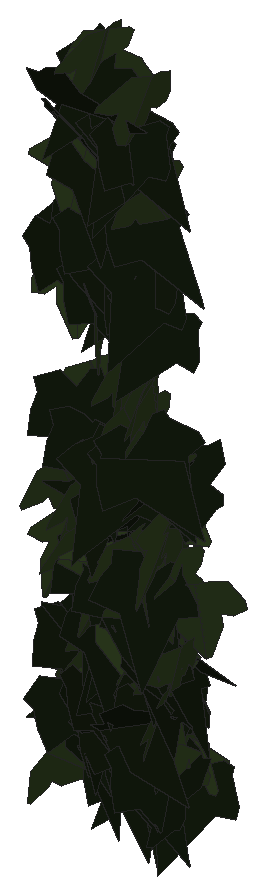
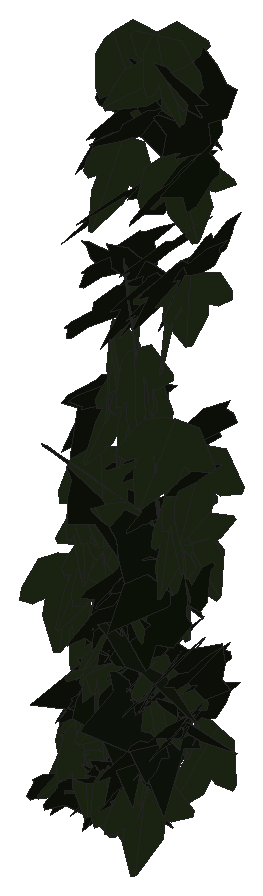
# SketchUp Ruby script. Lengths in inches.
U = 1.inch
M = Sketchup.active_model
def pt(a) = Geom::Point3d.new(a.map { |v| v * U })
def face(e, loops, mat)
  f = e.add_face(loops[0].map { |a| pt(a) })
  loops[1..].each { |l| e.add_face(l.map { |a| pt(a) }).erase! }
  f.material = f.back_material = mat if mat
  f
end
# faces: each face lists its corners as indices into pts; further lists are holes
def faces(e, pts, list, mat = nil) = list.each { |f| face(e, (f[0].is_a?(Array) ? f : [f]).map { |l| l.map { |i| pts[i] } }, mat) }
# xy, xz, yz: faces in a plane at the given z, y or x. An outline is a flat list of corners, or four numbers for a rectangle; further outlines are holes
def ring(l) = l.size == 4 ? [[l[0], l[1]], [l[2], l[1]], [l[2], l[3]], [l[0], l[3]]] : l.each_slice(2).to_a
def flat(e, list, mat, &to3) = list.each { |f| face(e, (f[0].is_a?(Array) ? f : [f]).map { |l| ring(l).map { |u, v| to3.(u, v) } }, mat) }
def xy(e, z, list, mat = nil) = flat(e, list, mat) { |x, y| [x, y, z] }
def xz(e, y, list, mat = nil) = flat(e, list, mat) { |x, z| [x, y, z] }
def yz(e, x, list, mat = nil) = flat(e, list, mat) { |y, z| [x, y, z] }
def lines(e, pts, list) = list.each { |a, b| e.add_line(pt(pts[a]), pt(pts[b])) }
# prism: a flat outline (further loops are holes) pulled along v
def prism(e, loops, v, mat = nil)
  f = face(e, loops, mat); d = Geom::Vector3d.new(v.map { |x| x * U })
  f.pushpull(f.normal.samedirection?(d) ? d.length : -d.length)
end
def box(e, o, s, mat = nil) = prism(e, [[o, [o[0] + s[0], o[1], o[2]], [o[0] + s[0], o[1] + s[1], o[2]], [o[0], o[1] + s[1], o[2]]]], [0, 0, s[2]], mat)
def at(x, y, z, deg = 0) = Geom::Transformation.translation(pt([x, y, z])) * Geom::Transformation.rotation(ORIGIN, Z_AXIS, deg.degrees)
def axes(o, x, y, z) = Geom::Transformation.new([*x, 0, *y, 0, *z, 0, *pt(o).to_a, 1])
def part(name) = M.definitions.add(name)
# library, detail: a bought-in or finely detailed component or shape, given as its bounding box
def library(name, o, s) = part(name).tap { |d| box(d.entities, o, s) }
def detail(e, o, s) = box(e.add_group.entities, o, s)
def put(e, d, t, mat = nil) = e.add_instance(d, t).tap { |i| i.material = mat if mat }
def group(e, t, mat = nil) = e.add_group.tap { |g| g.transformation = t; g.material = mat if mat }.entities
root = M.entities
M.materials.add("efeu1").color = [18, 25, 13]
M.materials.add("efeu2").color = [43, 57, 29]
c1 = part("ivyleaf_10")
p = [[0,0.5,-0.03],[-0.0625,2.02,-0.43],[-0.19,2.01,-0.46],[-0.54,1.05,-0.29],[-0.52,0.625,-0.18],[-0.83,0.76,-0.28],
  [-1.16,0.64,-0.33],[-1.15,0.33,-0.24],[-0.77,-0.39,0.02],[-0.3,-0.51,0.16],[0.04,-0.48,0.23],[-0.02,2.01,-0.4375],
  [-0.06,2.01,-0.43],[0.04,-0.49,0.23],[0.67,-0.49,0.14],[1.38,0.36,-0.2],[1.375,0.51,-0.24],[0.81,0.65,-0.19],
  [0.62,0.59,-0.15],[0.6,1.09,-0.28],[0.5,1.23,-0.31]]
faces(c1.entities,p,[[0,1,2,3,4,5,6,7,8,9,10],[11,12,0,13,14,15,16,17,18,19,20]],"efeu2")
c2 = part("ivyleaf_9")
p = [[1.54,2.16,1.25],[1.36,2.04,1.19],[-0.21,0.99,0.68],[-0.71,1.11,0.82],[-0.85,0.86,0.67],[-0.8,0.17,0.21],
  [-0.9,-0.01,0.1],[-0.67,-0.16,-0.02],[-0.08,-0.08,-0.05],[-0.03,-0.6,-0.4],[0.65,-0.88,-0.66],[0.83,-0.6,-0.49],
  [1.29,-0.42,-0.43],[1.8125,-0.07,-0.26],[1.21,0.44,0.15]]
faces(c2.entities,p,[[0,1,2,3,4,5,6,7,8,9,10,11,12,13,14]],"efeu1")
put(root,c1,axes([20.37,224.35,228.31],[-0.3494,-0.32143,-0.15685],[0.1692,0.04463,-0.46838],[0.31511,-0.38038,0.07758]))
put(root,c2,axes([20.24,224.07,224.83],[0.09687,-0.47627,-0.11741],[0.00815,0.12123,-0.48501],[0.49046,0.09205,0.03125]))
put(root,c1,axes([20.51,223.76,226.5],[-0.07022,-0.43594,0.23457],[0.0202,-0.23924,-0.43858],[0.49463,-0.05212,0.05121]))
put(root,c1,axes([20.48,224.17,224.74],[-0.14172,-0.41353,-0.24271],[0.081,0.2288,-0.43714],[0.4726,-0.16322,0.00214]))
put(root,c2,axes([20.35,223.5,230.78],[0.23139,-0.33588,-0.28921],[-0.15133,0.24678,-0.40767],[0.4166,0.2762,0.01255]))
put(root,c1,axes([20.49,224.22,224.48],[0.09238,-0.46179,0.16798],[0.05701,-0.1597,-0.47037],[0.48807,0.10606,0.02315]))
put(root,c2,axes([20.3,224.05,230.7],[0.17381,-0.40902,-0.22911],[-0.01366,0.23983,-0.43852],[0.46862,0.15869,0.07219]))
put(root,c2,axes([20.58,224.59,224.3],[-0.21746,0.3522,-0.28048],[-0.14101,0.24253,0.41388],[0.42758,0.2591,-0.00615]))
put(root,c1,axes([20.51,223.32,223.38],[-0.10609,-0.30973,-0.3779],[0.10594,0.36293,-0.3272],[0.47699,-0.14949,-0.01138]))
put(root,c2,axes([20.35,224.79,224.07],[0.13765,-0.4332,-0.2083],[-0.02684,0.2094,-0.45324],[0.47993,0.13596,0.03439]))
put(root,c1,axes([20.64,223.8,231.8125],[-0.40868,-0.25598,0.13211],[-0.04247,-0.17326,-0.4671],[0.28492,-0.39301,0.11987]))
put(root,c2,axes([20.33,224.31,223.98],[0.18097,-0.46436,-0.0403],[-0.01178,0.03866,-0.49836],[0.46595,0.18133,0.00305]))
put(root,c1,axes([20.45,223.8125,230.24],[0.33313,0.37278,0.00776],[0.01758,-0.00531,-0.49966],[-0.37245,0.33317,-0.01665]))
put(root,c2,axes([20.75,224.12,224.16],[-0.02358,0.49697,0.04962],[-0.06584,0.04615,-0.49349],[-0.49508,-0.02981,0.06327]))
put(root,c1,axes([20.58,223.96,226.91],[0.02594,-0.44996,-0.21648],[0.03553,0.21789,-0.44862],[0.49806,0.00789,0.04328]))
put(root,c1,axes([20.5625,223.4375,227.45],[-0.17095,-0.4291,-0.19144],[0.0823,0.17322,-0.46176],[0.4626,-0.18939,0.0114]))
put(root,c2,axes([20.24,223.74,232.21],[0.45361,-0.19536,0.07789],[0.07119,-0.03162,-0.49389],[0.1979,0.45917,-0.00087]))
put(root,c2,axes([20.41,223.91,228.28],[0.00995,-0.46863,-0.17403],[0.00475,0.17414,-0.46867],[0.49988,0.00767,0.00792]))
put(root,c1,axes([20.64,223.72,226.42],[-0.04724,-0.48873,-0.09438],[-0.00113,0.09491,-0.49091],[0.49776,-0.04616,-0.01007]))
put(root,c2,axes([20.91,224.5,225.26],[-0.3572,0.34232,0.07227],[-0.11607,-0.01851,-0.48599],[-0.33006,-0.36397,0.09269]))
put(root,c1,axes([20.58,224.55,223.09],[-0.20696,-0.45061,-0.06418],[0.09867,0.02441,-0.48956],[0.44433,-0.2153,0.07881]))
put(root,c2,axes([20.49,224.53,224.73],[-0.0751,-0.41377,0.27047],[0.0265,-0.27655,-0.41571],[0.49362,-0.04811,0.06347]))
put(root,c2,axes([20.49,223.97,224.48],[-0.27132,-0.05876,0.41585],[0.41678,0.02335,0.27522],[-0.05176,0.49599,0.03631]))
put(root,c1,axes([20.91,223.76,226.0625],[-0.37481,0.04297,0.32813],[-0.32819,0.01541,-0.3769],[-0.04251,-0.49791,0.01665]))
put(root,c1,axes([20.67,223.7,227.13],[0.03251,-0.48876,-0.10028],[0.00235,0.10064,-0.48976],[0.49894,0.03138,0.00884]))
put(root,c2,axes([20.43,223.63,224.24],[0.18742,-0.30232,-0.35139],[-0.02491,0.37191,-0.33326],[0.46287,0.14243,0.12434]))
put(root,c1,axes([20.67,224.16,223.99],[-0.04731,-0.44618,-0.22065],[0.05813,0.21518,-0.44757],[0.49435,-0.068,0.03151]))
put(root,c2,axes([20.98,224.29,224.21],[-0.46145,0.0104,0.19224],[-0.19219,-0.05385,-0.45843],[0.01117,-0.49698,0.0537]))
put(root,c1,axes([20.67,224.21,223.63],[-0.14099,0.47694,0.05148],[-0.01662,0.04877,-0.49734],[-0.47942,-0.14195,0.0021]))
put(root,c2,axes([20.7,223.67,226.21],[0.33201,0.33328,0.16938],[0.0305,0.20163,-0.45652],[-0.37261,0.31348,0.11355]))
put(root,c2,axes([20.52,224.02,223.69],[0.11665,-0.37629,0.3079],[0.07003,-0.30033,-0.39357],[0.48113,0.13495,-0.01736]))
put(root,c1,axes([20.82,224.12,228.08],[0.25588,-0.40065,-0.15494],[-0.04505,0.15432,-0.47345],[0.4272,0.25625,0.04287]))
put(root,c2,axes([20.63,224.02,227.25],[-0.01187,-0.49833,0.03913],[0.00498,-0.03925,-0.49843],[0.49983,-0.01144,0.00589]))
put(root,c1,axes([20.87,223.77,233.49],[-0.02101,-0.49705,0.05002],[-0.00449,-0.04987,-0.49749],[0.49954,-0.02135,-0.00237]))
put(root,c2,axes([20.73,224.39,224.29],[-0.0721,-0.28727,0.40284],[-0.04595,-0.40145,-0.2945],[0.49264,-0.07949,0.03149]))
put(root,c2,axes([20.5625,224.1,223.26],[0.16772,-0.44029,0.16738],[0.06501,-0.15434,-0.47112],[0.46652,0.1798,0.00547]))
put(root,c2,axes([20.48,224.47,225.39],[0.04296,-0.26879,0.41941],[0.32965,-0.30027,-0.2262],[0.37348,0.29596,0.15141]))
put(root,c2,axes([20.65,223.95,231.72],[0.05413,-0.49542,0.04041],[0.00599,-0.03999,-0.49836],[0.49703,0.05444,0.0016]))
put(root,c1,axes([20.85,224.18,225.84],[0.03531,-0.3953,0.30413],[0.03242,-0.30243,-0.39685],[0.4977,0.04775,0.00427]))
put(root,c2,axes([21,224,226.72],[-0.20226,0.37172,-0.2663],[0.07528,-0.26015,-0.42031],[-0.45103,-0.21012,0.04926]))
put(root,c2,axes([20.42,223.55,232.55],[0.21336,-0.14445,0.4285],[0.38311,-0.19395,-0.25614],[0.24021,0.43763,0.02792]))
put(root,c1,axes([20.87,224.42,223.56],[-0.16519,-0.38909,0.26706],[0.05455,-0.29679,-0.39867],[0.46876,-0.10258,0.14051]))
put(root,c2,axes([21.01,223.81,233.125],[-0.49336,-0.03735,-0.07213],[0.07153,0.01069,-0.49474],[0.0385,-0.49849,-0.0052]))
put(root,c2,axes([20.67,223.89,227.86],[0.02573,-0.48529,-0.11761],[0.02555,0.11889,-0.48499],[0.49868,0.01895,0.03092]))
put(root,c2,axes([21.09,224.46,224.24],[-0.06834,0.48357,0.10721],[-0.09359,0.09367,-0.48215],[-0.48638,-0.08597,0.07772]))
put(root,c2,axes([20.66,224.15,224.9375],[0.06793,-0.48441,0.10358],[0.03214,-0.10002,-0.48884],[0.49432,0.07307,0.01755]))
put(root,c1,axes([20.99,223.49,229.74],[0.25919,-0.21531,-0.36941],[-0.09196,0.3938,-0.29405],[0.41757,0.22037,0.16454]))
put(root,c2,axes([20.96,224.53,224.24],[-0.36276,-0.34401,-0.00803],[0.03886,-0.02936,-0.49762],[0.3419,-0.36166,0.04804]))
put(root,c2,axes([20.78,223.93,226.1875],[-0.00579,-0.4539,-0.20962],[0.00542,0.20957,-0.45393],[0.49994,-0.00753,0.00249]))
put(root,c2,axes([20.7,223.88,230.82],[0.1826,-0.43591,-0.16323],[0.04546,0.1912,-0.45976],[0.46324,0.15306,0.10946]))
put(root,c1,axes([21.05,224.48,223.17],[-0.10931,-0.48062,0.08399],[0.00011,-0.0861,-0.49253],[0.4879,-0.10766,0.01893]))
put(root,c1,axes([21.04,223.92,228.49],[0.25796,-0.39127,-0.17426],[-0.02284,0.19056,-0.4617],[0.42771,0.24616,0.08045]))
put(root,c1,axes([20.74,223.73,233.24],[0.20707,0.10486,0.44286],[0.25553,0.37583,-0.20846],[-0.3766,0.31266,0.10206]))
put(root,c1,axes([20.87,224.42,224.55],[-0.32306,-0.20575,-0.3214],[0.28718,0.14623,-0.38229],[0.25131,-0.4316,0.0237]))
put(root,c2,axes([20.72,224.15,225.28],[0.22031,-0.36683,0.25864],[0.13,-0.22362,-0.4279],[0.4296,0.25579,-0.00315]))
put(root,c1,axes([21.14,224.08,224.4],[0.22301,0.42446,0.14178],[-0.10061,-0.1068,0.47799],[0.43606,-0.24172,0.03778]))
put(root,c2,axes([20.87,224.39,223.13],[0.0635,-0.49132,-0.06759],[0.00124,0.0683,-0.49531],[0.49595,0.06274,0.0099]))
put(root,c2,axes([20.82,223.71,230.17],[0.21822,-0.42669,-0.14253],[-0.0073,0.15504,-0.4753],[0.44981,0.20952,0.06143]))
put(root,c2,axes([20.84,223.62,224.38],[0.2711,-0.40497,-0.11183],[-0.04738,0.10278,-0.48702],[0.41745,0.27466,0.01735]))
put(root,c2,axes([20.85,223.91,230.26],[0.18674,-0.38863,-0.25316],[-0.02705,0.26332,-0.42418],[0.46303,0.17212,0.07732]))
put(root,c1,axes([21.27,224.02,226.04],[-0.00844,0.16666,0.47133],[-0.20814,-0.42977,0.14824],[0.45454,-0.1937,0.07663]))
put(root,c1,axes([21.11,224.04,228.91],[0.0227,-0.48798,-0.1066],[0.01953,0.1075,-0.48792],[0.4991,0.01799,0.02394]))
put(root,c2,axes([21.3,224.61,223.29],[-0.48046,-0.13743,-0.01638],[0.02862,-0.04075,-0.49751],[0.13541,-0.47901,0.04703]))
put(root,c2,axes([20.92,223.96,223.52],[0.40036,-0.2295,-0.19247],[-0.07372,0.23591,-0.43464],[0.29031,0.3764,0.15506]))
put(root,c1,axes([21.25,224.29,224.74],[-0.35844,-0.33326,0.10228],[-0.03058,-0.11608,-0.48538],[0.34726,-0.35421,0.06283]))
put(root,c2,axes([20.98,224.09,223.4],[0.07741,-0.35267,-0.34588],[0.00667,0.35082,-0.3562],[0.49393,0.05053,0.05902]))
put(root,c2,axes([20.84,224.46,224.79],[0.45182,-0.04789,0.20872],[0.21007,0.00459,-0.45371],[0.04154,0.49768,0.02427]))
put(root,c2,axes([21.24,223.85,227.51],[-0.25376,-0.41665,0.10957],[-0.03334,-0.10778,-0.4871],[0.42952,-0.25453,0.02692]))
put(root,c1,axes([21.31,224.4375,224.66],[-0.02024,-0.49954,0.00703],[-0.00053,-0.00701,-0.49995],[0.49959,-0.02025,-0.00024]))
put(root,c1,axes([21.29,223.96,230.14],[0.22659,-0.43826,-0.08116],[0.00418,0.09313,-0.49123],[0.44569,0.22194,0.04586]))
put(root,c2,axes([21.14,224.32,224.63],[-0.29176,-0.20649,-0.34963],[0.28524,0.20219,-0.35743],[0.28899,-0.40802,-0.00019]))
put(root,c2,axes([21.1,224.0625,225.96],[0.0671,-0.39062,-0.30482],[0.01045,0.30865,-0.39322],[0.49537,0.0464,0.04959]))
put(root,c2,axes([21.12,223.9,225.91],[0.03092,-0.48932,-0.09803],[0.012,0.09892,-0.48997],[0.4989,0.02795,0.01786]))
put(root,c1,axes([21.34,224.32,224.47],[0.08833,-0.45758,-0.18115],[-0.01063,0.18223,-0.46549],[0.49202,0.08609,0.02247]))
put(root,c1,axes([21.09,224.5,224.42],[-0.36196,-0.07032,-0.3377],[0.34006,0.00925,-0.36643],[0.05778,-0.49494,0.04113]))
put(root,c2,axes([21.47,224.08,230.48],[-0.47898,-0.13047,-0.0596],[0.06933,-0.02872,-0.49434],[0.12557,-0.48182,0.04561]))
put(root,c1,axes([21.375,223.67,228.39],[-0.05484,-0.42646,-0.2552],[0.0419,0.25186,-0.42989],[0.49521,-0.06854,0.00812]))
put(root,c2,axes([21.25,224.57,224.47],[-0.10606,-0.48862,-0.00073],[0.00014,0.00071,-0.5],[0.48862,-0.10606,-0.00002]))
put(root,c1,axes([21.49,224.32,224.29],[-0.09872,-0.45704,0.17711],[-0.04053,-0.17243,-0.46757],[0.48848,-0.10668,-0.003]))
put(root,c1,axes([21.42,223.76,226.51],[-0.20997,-0.41383,-0.18617],[0.07456,0.17088,-0.46394],[0.44761,-0.22259,-0.01006]))
put(root,c1,axes([21.42,224.34,226.76],[0.41391,0.2473,-0.13236],[-0.12128,-0.05496,-0.48195],[-0.25292,0.43107,0.01449]))
put(root,c2,axes([21.18,224.18,223.59],[0.13961,-0.45608,0.15001],[0.06183,-0.13784,-0.47663],[0.47612,0.15164,0.01791]))
put(root,c2,axes([21.42,223.94,232.23],[-0.23092,-0.40464,0.18151],[-0.00059,-0.20436,-0.45633],[0.44348,-0.21096,0.09391]))
put(root,c2,axes([21.61,224.07,227.21],[-0.12448,0.4523,-0.173],[0.05532,-0.16417,-0.46903],[-0.48109,-0.13591,-0.00917]))
put(root,c1,axes([21.52,224.15,223.86],[0.46931,-0.05826,-0.16233],[-0.13794,0.1557,-0.45468],[0.10353,0.47155,0.13007]))
put(root,c2,axes([21.31,224.1,223.64],[-0.01831,-0.2072,-0.45468],[0.02045,0.45429,-0.20785],[0.49925,-0.02621,-0.00816]))
put(root,c2,axes([21.31,224.26,225.5],[0.01562,-0.49709,-0.05151],[-0.00092,0.0515,-0.49734],[0.49976,0.01563,0.0007]))
put(root,c1,axes([21.55,224.22,227.41],[-0.30199,-0.39847,0.00448],[0.00262,-0.0076,-0.49994],[0.39849,-0.30193,0.00668]))
put(root,c1,axes([21.51,224.52,223.24],[0.48047,0.07601,-0.11564],[-0.12257,0.03977,-0.48311],[-0.06425,0.49259,0.05685]))
put(root,c2,axes([21.41,224.62,223.12],[-0.16968,-0.46727,-0.05356],[0.02119,0.04929,-0.49711],[0.46985,-0.17098,0.00308]))
put(root,c1,axes([21.52,224.58,223.65],[-0.0762,-0.49303,-0.03332],[0.03406,0.0284,-0.49803],[0.49298,-0.07817,0.02926]))
put(root,c1,axes([21.55,224.3,223.34],[-0.18742,-0.46084,0.04997],[0.00713,-0.05676,-0.49672],[0.46349,-0.18548,0.02785]))
put(root,c2,axes([21.56,223.67,232.52],[-0.44462,-0.16102,-0.16244],[0.15397,0.05189,-0.47286],[0.16914,-0.47051,0.00344]))
put(root,c2,axes([21.36,223.35,224.08],[0.41255,0.25565,0.12018],[0.0948,0.07509,-0.48515],[-0.26611,0.42309,0.01349]))
put(root,c1,axes([21.49,224.22,224.99],[-0.17926,0.46437,-0.04723],[0.02184,-0.0422,-0.49774],[-0.46625,-0.18051,-0.00515]))
put(root,c2,axes([21.3125,224.19,224.99],[0.09404,-0.4248,0.24638],[0.06872,-0.23701,-0.43486],[0.48625,0.11565,0.0138]))
put(root,c1,axes([21.66,223.94,225.82],[-0.21847,-0.44925,0.02116],[-0.00618,-0.02052,-0.49954],[0.4497,-0.21853,0.00341]))
put(root,c2,axes([21.47,224.42,224.26],[-0.03394,-0.49465,0.06454],[-0.01392,-0.06373,-0.49573],[0.49865,-0.03544,-0.00945]))
put(root,c1,axes([21.69,223.65,233.16],[-0.07566,-0.48427,0.09879],[-0.02629,-0.09585,-0.49002],[0.49354,-0.07934,-0.01096]))
put(root,c1,axes([21.65,223.85,225.98],[-0.16989,0.43174,0.18639],[-0.09111,0.16421,-0.4634],[-0.46134,-0.19142,0.02287]))
put(root,c2,axes([21.58,223.93,230.34],[-0.16521,-0.44582,0.15475],[-0.02718,-0.1547,-0.47469],[0.47113,-0.16526,0.02688]))
put(root,c2,axes([21.43,223.68,232.45],[0.19136,-0.39542,-0.23879],[-0.01698,0.25228,-0.43136],[0.46162,0.1732,0.08312]))
put(root,c1,axes([21.65,223.7,228.23],[-0.01076,-0.31975,-0.38425],[0.06976,0.37961,-0.31785],[0.49499,-0.06046,0.03644]))
put(root,c1,axes([21.66,223.71,231.69],[-0.12549,-0.39912,-0.27378],[0.07777,0.26253,-0.41837],[0.47771,-0.14758,-0.00381]))
put(root,c1,axes([21.53,224.2,223.3],[-0.02233,-0.20575,-0.45516],[0.25556,0.38676,-0.18737],[0.42917,-0.24101,0.08789]))
put(root,c1,axes([21.72,223.65,228.85],[0.19323,-0.45362,-0.08299],[-0.0143,0.08404,-0.49268],[0.46093,0.19278,0.01951]))
put(root,c2,axes([21.65,224.21,229.67],[-0.18562,-0.41002,0.21778],[-0.04756,-0.21652,-0.44817],[0.46183,-0.18709,0.04138]))
put(root,c2,axes([21.39,223.45,224.2],[-0.0585,-0.17367,-0.46521],[0.30494,0.35713,-0.17167],[0.39191,-0.3038,0.06413]))
put(root,c2,axes([21.45,224.54,224.625],[0.23561,-0.43884,0.04369],[0.01152,-0.04339,-0.49798],[0.44086,0.23567,-0.01034]))
put(root,c2,axes([21.45,223.81,231.26],[0.22099,-0.41081,-0.17999],[0.04995,0.22195,-0.44525],[0.44572,0.17881,0.13914]))
put(root,c1,axes([21.75,223.67,228.95],[0.15179,-0.41834,-0.22793],[0.00147,0.23963,-0.43883],[0.4764,0.13255,0.07398]))
put(root,c1,axes([21.85,223.9,223.5625],[-0.41057,-0.26221,0.11262],[-0.08058,-0.08277,-0.48647],[0.27376,-0.41761,0.0257]))
put(root,c1,axes([21.83,224.21,226.8],[0.04262,-0.47949,-0.13518],[-0.00789,0.13501,-0.48136],[0.49812,0.04317,0.00395]))
put(root,c1,axes([21.87,224.04,224.88],[0.00173,-0.49898,0.03182],[0.01047,-0.03177,-0.49888],[0.49989,0.00239,0.01034]))
put(root,c2,axes([21.72,223.75,226.14],[-0.09893,-0.48818,-0.04356],[0.00738,0.04295,-0.4981],[0.49006,-0.0992,-0.00129]))
put(root,c1,axes([21.84,223.78,224.37],[0.2349,-0.44005,0.03434],[0.01539,-0.03072,-0.49882],[0.44112,0.2354,-0.00089]))
put(root,c2,axes([21.63,223.67,223.54],[0.19252,-0.42495,-0.17987],[-0.04121,0.17829,-0.46531],[0.4596,0.19399,0.03363]))
put(root,c1,axes([21.83,224.08,225.98],[-0.02837,-0.37295,-0.33182],[0.09013,0.32307,-0.37082],[0.49099,-0.08085,0.0489]))
put(root,c2,axes([22.16,224.27,227.38],[-0.47527,0.13257,0.08087],[-0.1026,-0.07258,-0.48395],[-0.11657,-0.47661,0.0962]))
put(root,c2,axes([21.82,224.57,223.07],[-0.23192,-0.44094,0.04226],[0.00572,-0.05067,-0.49739],[0.44292,-0.23023,0.02854]))
put(root,c2,axes([22.25,223.7,223.18],[-0.29128,0.33475,0.23042],[-0.17671,0.15097,-0.4427],[-0.36597,-0.33933,0.03036]))
put(root,c1,axes([21.84,223.85,226.8],[0.11564,-0.37814,0.306],[0.1292,-0.27935,-0.39404],[0.46897,0.1702,0.0331]))
put(root,c2,axes([21.75,223.56,228.21],[-0.01791,-0.36221,-0.34422],[0.07065,0.33914,-0.36054],[0.49466,-0.06156,0.03903]))
put(root,c2,axes([21.7,223.48,228.14],[0.06948,-0.35556,-0.3446],[0.10247,0.35077,-0.34127],[0.48443,-0.0232,0.12162]))
put(root,c2,axes([21.66,223.9,224.6],[0.09857,-0.39901,0.28473],[0.14865,-0.25242,-0.4052],[0.4671,0.16453,0.06887]))
put(root,c1,axes([22.03,224.29,225.74],[-0.39011,-0.31049,-0.0376],[0.02704,0.02641,-0.49857],[0.31158,-0.39103,-0.00382]))
